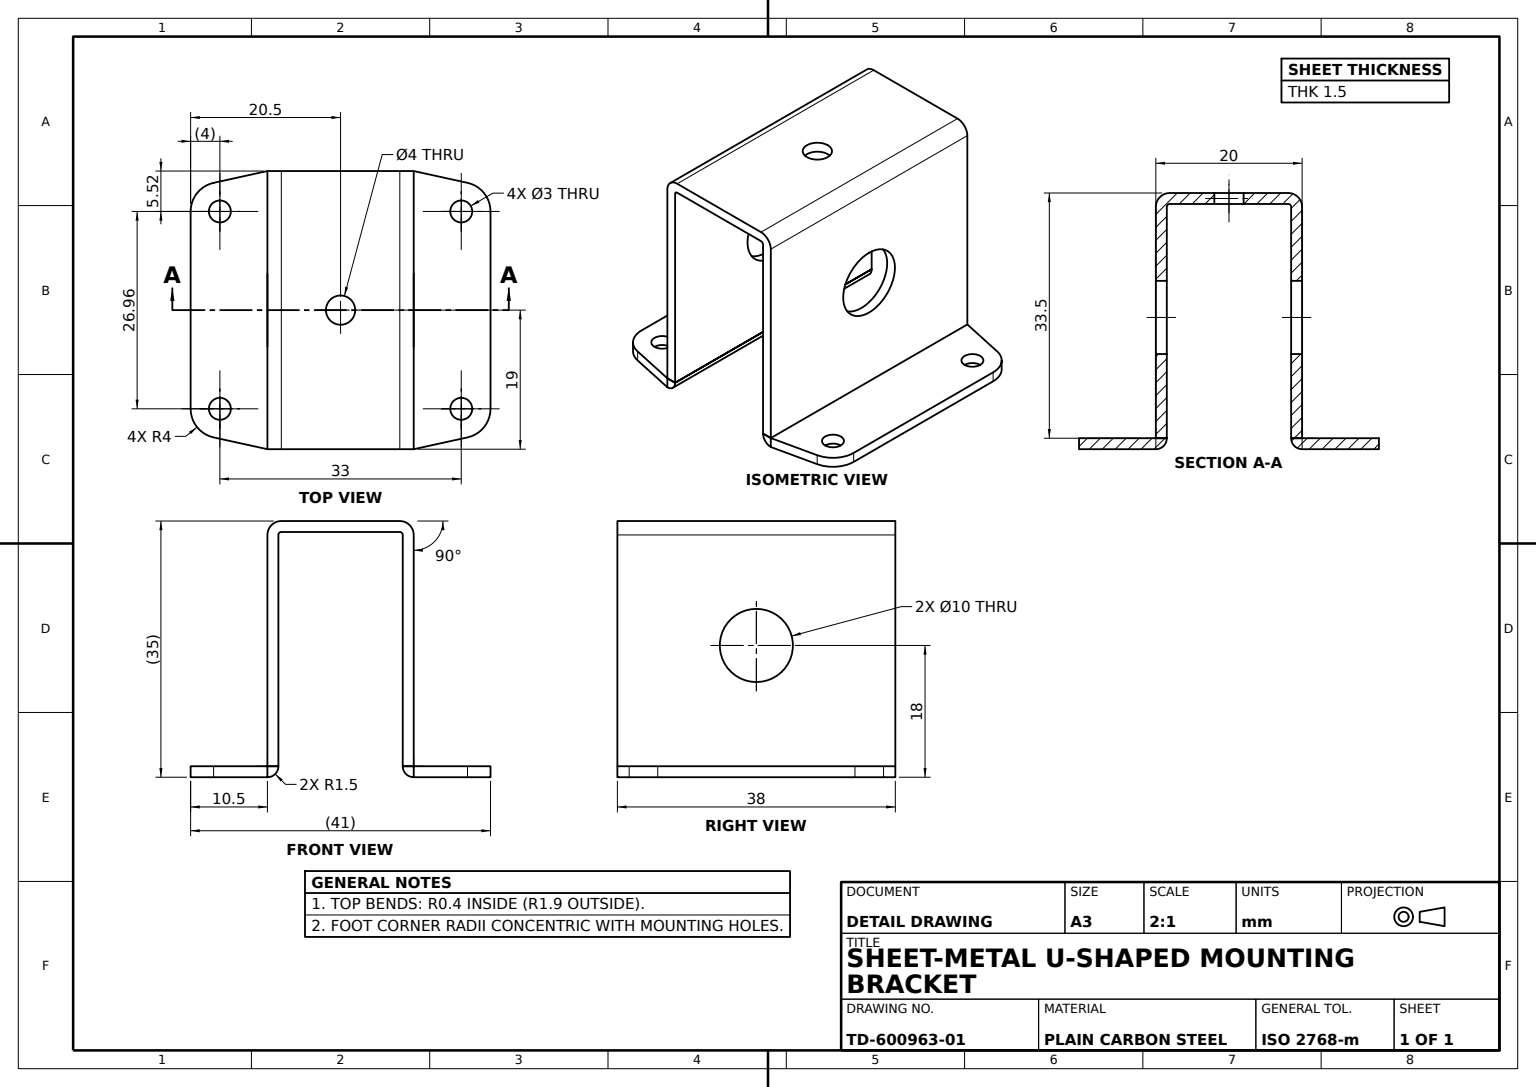
ISO-10303-21;
HEADER;
FILE_DESCRIPTION((''),'2;1');
FILE_NAME('','',(''),(''),'','','');
FILE_SCHEMA(('AUTOMOTIVE_DESIGN'));
ENDSEC;
DATA;
#1=APPLICATION_CONTEXT('');
#2=PRODUCT_CONTEXT('',#1,'mechanical');
#3=PRODUCT('','','',(#2));
#4=PRODUCT_DEFINITION_FORMATION('','',#3);
#5=PRODUCT_DEFINITION_CONTEXT('',#1,'design');
#6=PRODUCT_DEFINITION('','',#4,#5);
#7=PRODUCT_DEFINITION_SHAPE('','',#6);
#8=(LENGTH_UNIT()NAMED_UNIT(*)SI_UNIT(.MILLI.,.METRE.));
#9=(NAMED_UNIT(*)PLANE_ANGLE_UNIT()SI_UNIT($,.RADIAN.));
#10=(NAMED_UNIT(*)SI_UNIT($,.STERADIAN.)SOLID_ANGLE_UNIT());
#11=UNCERTAINTY_MEASURE_WITH_UNIT(LENGTH_MEASURE(1.E-05),#8,'distance_accuracy_value','');
#12=(GEOMETRIC_REPRESENTATION_CONTEXT(3)GLOBAL_UNCERTAINTY_ASSIGNED_CONTEXT((#11))GLOBAL_UNIT_ASSIGNED_CONTEXT((#8,#9,#10))REPRESENTATION_CONTEXT('',''));
#13=CARTESIAN_POINT('',(-15.,-33.5,13.481351));
#14=VERTEX_POINT('',#13);
#15=CARTESIAN_POINT('',(-18.,-33.5,13.481351));
#16=VERTEX_POINT('',#15);
#17=CARTESIAN_POINT('',(-16.5,-33.5,13.481351));
#18=DIRECTION('',(0.,-1.,0.));
#19=DIRECTION('',(1.,0.,0.));
#20=AXIS2_PLACEMENT_3D('',#17,#18,#19);
#21=CIRCLE('',#20,1.5);
#22=EDGE_CURVE('',#14,#16,#21,.T.);
#23=ORIENTED_EDGE('',*,*,#22,.F.);
#24=CARTESIAN_POINT('',(-15.,-35.,13.481351));
#25=VERTEX_POINT('',#24);
#26=DIRECTION('',(0.,1.,0.));
#27=VECTOR('',#26,1000.);
#28=LINE('',#24,#27);
#29=EDGE_CURVE('',#25,#14,#28,.T.);
#30=ORIENTED_EDGE('',*,*,#29,.F.);
#31=CARTESIAN_POINT('',(-18.,-35.,13.481351));
#32=VERTEX_POINT('',#31);
#33=CARTESIAN_POINT('',(-16.5,-35.,13.481351));
#34=AXIS2_PLACEMENT_3D('',#33,#18,#19);
#35=CIRCLE('',#34,1.5);
#36=EDGE_CURVE('',#25,#32,#35,.T.);
#37=ORIENTED_EDGE('',*,*,#36,.T.);
#38=LINE('',#31,#27);
#39=EDGE_CURVE('',#32,#16,#38,.T.);
#40=ORIENTED_EDGE('',*,*,#39,.T.);
#41=EDGE_LOOP('',(#23,#30,#37,#40));
#42=FACE_OUTER_BOUND('',#41,.T.);
#43=DIRECTION('',(-1.,0.,0.));
#44=AXIS2_PLACEMENT_3D('',#33,#26,#43);
#45=CYLINDRICAL_SURFACE('',#44,1.5);
#46=ADVANCED_FACE('',(#42),#45,.F.);
#47=CARTESIAN_POINT('',(-10.,-35.,19.));
#48=VERTEX_POINT('',#47);
#49=CARTESIAN_POINT('',(-10.,-33.5,19.));
#50=VERTEX_POINT('',#49);
#51=LINE('',#47,#27);
#52=EDGE_CURVE('',#48,#50,#51,.T.);
#53=ORIENTED_EDGE('',*,*,#52,.F.);
#54=CARTESIAN_POINT('',(-8.5,-33.5,19.));
#55=VERTEX_POINT('',#54);
#56=DIRECTION('',(0.,0.,1.));
#57=AXIS2_PLACEMENT_3D('',#49,#56,#26);
#58=CIRCLE('',#57,1.5);
#59=EDGE_CURVE('',#48,#55,#58,.T.);
#60=ORIENTED_EDGE('',*,*,#59,.T.);
#61=VECTOR('',#43,1000.);
#62=LINE('',#49,#61);
#63=EDGE_CURVE('',#55,#50,#62,.T.);
#64=ORIENTED_EDGE('',*,*,#63,.T.);
#65=EDGE_LOOP('',(#53,#60,#64));
#66=FACE_OUTER_BOUND('',#65,.T.);
#67=DIRECTION('',(0.,0.,-1.));
#68=AXIS2_PLACEMENT_3D('',#47,#67,#26);
#69=PLANE('',#68);
#70=ADVANCED_FACE('',(#66),#69,.F.);
#71=CARTESIAN_POINT('',(-17.355897,-35.,-17.388708));
#72=VERTEX_POINT('',#71);
#73=CARTESIAN_POINT('',(-17.355897,-33.5,-17.388708));
#74=VERTEX_POINT('',#73);
#75=LINE('',#71,#27);
#76=EDGE_CURVE('',#72,#74,#75,.T.);
#77=ORIENTED_EDGE('',*,*,#76,.F.);
#78=CARTESIAN_POINT('',(-20.5,-35.,-13.481351));
#79=VERTEX_POINT('',#78);
#80=CARTESIAN_POINT('',(-16.5,-35.,-13.481351));
#81=AXIS2_PLACEMENT_3D('',#80,#18,#19);
#82=CIRCLE('',#81,4.);
#83=EDGE_CURVE('',#79,#72,#82,.T.);
#84=ORIENTED_EDGE('',*,*,#83,.F.);
#85=CARTESIAN_POINT('',(-20.5,-33.5,-13.481351));
#86=VERTEX_POINT('',#85);
#87=LINE('',#78,#27);
#88=EDGE_CURVE('',#79,#86,#87,.T.);
#89=ORIENTED_EDGE('',*,*,#88,.T.);
#90=CARTESIAN_POINT('',(-16.5,-33.5,-13.481351));
#91=AXIS2_PLACEMENT_3D('',#90,#18,#19);
#92=CIRCLE('',#91,4.);
#93=EDGE_CURVE('',#86,#74,#92,.T.);
#94=ORIENTED_EDGE('',*,*,#93,.T.);
#95=EDGE_LOOP('',(#77,#84,#89,#94));
#96=FACE_OUTER_BOUND('',#95,.T.);
#97=AXIS2_PLACEMENT_3D('',#80,#26,#43);
#98=CYLINDRICAL_SURFACE('',#97,4.);
#99=ADVANCED_FACE('',(#96),#98,.T.);
#100=CARTESIAN_POINT('',(-18.,-33.5,-13.481351));
#101=VERTEX_POINT('',#100);
#102=CARTESIAN_POINT('',(-15.,-33.5,-13.481351));
#103=VERTEX_POINT('',#102);
#104=CIRCLE('',#91,1.5);
#105=EDGE_CURVE('',#101,#103,#104,.T.);
#106=ORIENTED_EDGE('',*,*,#105,.T.);
#107=EDGE_CURVE('',#103,#101,#104,.T.);
#108=ORIENTED_EDGE('',*,*,#107,.T.);
#109=EDGE_LOOP('',(#106,#108));
#110=FACE_BOUND('',#109,.T.);
#111=EDGE_CURVE('',#16,#14,#21,.T.);
#112=ORIENTED_EDGE('',*,*,#111,.T.);
#113=ORIENTED_EDGE('',*,*,#22,.T.);
#114=EDGE_LOOP('',(#112,#113));
#115=FACE_BOUND('',#114,.T.);
#116=CARTESIAN_POINT('',(-20.5,-33.5,13.481351));
#117=VERTEX_POINT('',#116);
#118=VECTOR('',#67,1000.);
#119=LINE('',#116,#118);
#120=EDGE_CURVE('',#117,#86,#119,.T.);
#121=ORIENTED_EDGE('',*,*,#120,.F.);
#122=CARTESIAN_POINT('',(-17.355897,-33.5,17.388708));
#123=VERTEX_POINT('',#122);
#124=AXIS2_PLACEMENT_3D('',#17,#18,#43);
#125=CIRCLE('',#124,4.);
#126=EDGE_CURVE('',#123,#117,#125,.T.);
#127=ORIENTED_EDGE('',*,*,#126,.F.);
#128=DIRECTION('',(-0.976839286,0.,-0.21397432));
#129=VECTOR('',#128,1000.);
#130=LINE('',#49,#129);
#131=EDGE_CURVE('',#50,#123,#130,.T.);
#132=ORIENTED_EDGE('',*,*,#131,.F.);
#133=ORIENTED_EDGE('',*,*,#63,.F.);
#134=CARTESIAN_POINT('',(-8.5,-33.5,-19.));
#135=VERTEX_POINT('',#134);
#136=VECTOR('',#56,1000.);
#137=LINE('',#54,#136);
#138=EDGE_CURVE('',#135,#55,#137,.T.);
#139=ORIENTED_EDGE('',*,*,#138,.F.);
#140=CARTESIAN_POINT('',(-10.,-33.5,-19.));
#141=VERTEX_POINT('',#140);
#142=VECTOR('',#19,1000.);
#143=LINE('',#140,#142);
#144=EDGE_CURVE('',#141,#135,#143,.T.);
#145=ORIENTED_EDGE('',*,*,#144,.F.);
#146=DIRECTION('',(0.976839286,0.,-0.21397432));
#147=VECTOR('',#146,1000.);
#148=LINE('',#73,#147);
#149=EDGE_CURVE('',#74,#141,#148,.T.);
#150=ORIENTED_EDGE('',*,*,#149,.F.);
#151=ORIENTED_EDGE('',*,*,#93,.F.);
#152=EDGE_LOOP('',(#121,#127,#132,#133,#139,#145,#150,#151));
#153=FACE_OUTER_BOUND('',#152,.T.);
#154=PLANE('',#91);
#155=ADVANCED_FACE('',(#110,#115,#153),#154,.F.);
#156=ORIENTED_EDGE('',*,*,#52,.T.);
#157=ORIENTED_EDGE('',*,*,#131,.T.);
#158=CARTESIAN_POINT('',(-17.355897,-35.,17.388708));
#159=VERTEX_POINT('',#158);
#160=LINE('',#158,#27);
#161=EDGE_CURVE('',#159,#123,#160,.T.);
#162=ORIENTED_EDGE('',*,*,#161,.F.);
#163=LINE('',#47,#129);
#164=EDGE_CURVE('',#48,#159,#163,.T.);
#165=ORIENTED_EDGE('',*,*,#164,.F.);
#166=EDGE_LOOP('',(#156,#157,#162,#165));
#167=FACE_OUTER_BOUND('',#166,.T.);
#168=DIRECTION('',(0.21397432,0.,-0.976839286));
#169=AXIS2_PLACEMENT_3D('',#47,#168,#128);
#170=PLANE('',#169);
#171=ADVANCED_FACE('',(#167),#170,.F.);
#172=ORIENTED_EDGE('',*,*,#138,.T.);
#173=ORIENTED_EDGE('',*,*,#59,.F.);
#174=CARTESIAN_POINT('',(-10.,-35.,-19.));
#175=VERTEX_POINT('',#174);
#176=LINE('',#47,#136);
#177=EDGE_CURVE('',#175,#48,#176,.T.);
#178=ORIENTED_EDGE('',*,*,#177,.F.);
#179=AXIS2_PLACEMENT_3D('',#140,#67,#18);
#180=CIRCLE('',#179,1.5);
#181=EDGE_CURVE('',#135,#175,#180,.T.);
#182=ORIENTED_EDGE('',*,*,#181,.F.);
#183=EDGE_LOOP('',(#172,#173,#178,#182));
#184=FACE_OUTER_BOUND('',#183,.T.);
#185=CARTESIAN_POINT('',(-10.,-33.5,-13.481351));
#186=AXIS2_PLACEMENT_3D('',#185,#67,#26);
#187=CYLINDRICAL_SURFACE('',#186,1.5);
#188=ADVANCED_FACE('',(#184),#187,.T.);
#189=ORIENTED_EDGE('',*,*,#161,.T.);
#190=ORIENTED_EDGE('',*,*,#126,.T.);
#191=CARTESIAN_POINT('',(-20.5,-35.,13.481351));
#192=VERTEX_POINT('',#191);
#193=LINE('',#191,#27);
#194=EDGE_CURVE('',#192,#117,#193,.T.);
#195=ORIENTED_EDGE('',*,*,#194,.F.);
#196=AXIS2_PLACEMENT_3D('',#33,#18,#43);
#197=CIRCLE('',#196,4.);
#198=EDGE_CURVE('',#159,#192,#197,.T.);
#199=ORIENTED_EDGE('',*,*,#198,.F.);
#200=EDGE_LOOP('',(#189,#190,#195,#199));
#201=FACE_OUTER_BOUND('',#200,.T.);
#202=CYLINDRICAL_SURFACE('',#44,4.);
#203=ADVANCED_FACE('',(#201),#202,.T.);
#204=ORIENTED_EDGE('',*,*,#144,.T.);
#205=ORIENTED_EDGE('',*,*,#181,.T.);
#206=LINE('',#174,#27);
#207=EDGE_CURVE('',#175,#141,#206,.T.);
#208=ORIENTED_EDGE('',*,*,#207,.T.);
#209=EDGE_LOOP('',(#204,#205,#208));
#210=FACE_OUTER_BOUND('',#209,.T.);
#211=AXIS2_PLACEMENT_3D('',#174,#56,#18);
#212=PLANE('',#211);
#213=ADVANCED_FACE('',(#210),#212,.F.);
#214=LINE('',#71,#147);
#215=EDGE_CURVE('',#72,#175,#214,.T.);
#216=ORIENTED_EDGE('',*,*,#215,.F.);
#217=ORIENTED_EDGE('',*,*,#76,.T.);
#218=ORIENTED_EDGE('',*,*,#149,.T.);
#219=ORIENTED_EDGE('',*,*,#207,.F.);
#220=EDGE_LOOP('',(#216,#217,#218,#219));
#221=FACE_OUTER_BOUND('',#220,.T.);
#222=DIRECTION('',(0.21397432,0.,0.976839286));
#223=AXIS2_PLACEMENT_3D('',#71,#222,#146);
#224=PLANE('',#223);
#225=ADVANCED_FACE('',(#221),#224,.F.);
#226=ORIENTED_EDGE('',*,*,#29,.T.);
#227=ORIENTED_EDGE('',*,*,#111,.F.);
#228=ORIENTED_EDGE('',*,*,#39,.F.);
#229=EDGE_CURVE('',#32,#25,#35,.T.);
#230=ORIENTED_EDGE('',*,*,#229,.T.);
#231=EDGE_LOOP('',(#226,#227,#228,#230));
#232=FACE_OUTER_BOUND('',#231,.T.);
#233=ADVANCED_FACE('',(#232),#45,.F.);
#234=ORIENTED_EDGE('',*,*,#120,.T.);
#235=ORIENTED_EDGE('',*,*,#88,.F.);
#236=LINE('',#191,#118);
#237=EDGE_CURVE('',#192,#79,#236,.T.);
#238=ORIENTED_EDGE('',*,*,#237,.F.);
#239=ORIENTED_EDGE('',*,*,#194,.T.);
#240=EDGE_LOOP('',(#234,#235,#238,#239));
#241=FACE_OUTER_BOUND('',#240,.T.);
#242=AXIS2_PLACEMENT_3D('',#191,#19,#26);
#243=PLANE('',#242);
#244=ADVANCED_FACE('',(#241),#243,.F.);
#245=ORIENTED_EDGE('',*,*,#105,.F.);
#246=CARTESIAN_POINT('',(-18.,-35.,-13.481351));
#247=VERTEX_POINT('',#246);
#248=LINE('',#246,#27);
#249=EDGE_CURVE('',#247,#101,#248,.T.);
#250=ORIENTED_EDGE('',*,*,#249,.F.);
#251=CARTESIAN_POINT('',(-15.,-35.,-13.481351));
#252=VERTEX_POINT('',#251);
#253=CIRCLE('',#81,1.5);
#254=EDGE_CURVE('',#247,#252,#253,.T.);
#255=ORIENTED_EDGE('',*,*,#254,.T.);
#256=LINE('',#251,#27);
#257=EDGE_CURVE('',#252,#103,#256,.T.);
#258=ORIENTED_EDGE('',*,*,#257,.T.);
#259=EDGE_LOOP('',(#245,#250,#255,#258));
#260=FACE_OUTER_BOUND('',#259,.T.);
#261=CYLINDRICAL_SURFACE('',#97,1.5);
#262=ADVANCED_FACE('',(#260),#261,.F.);
#263=ORIENTED_EDGE('',*,*,#257,.F.);
#264=EDGE_CURVE('',#252,#247,#253,.T.);
#265=ORIENTED_EDGE('',*,*,#264,.T.);
#266=ORIENTED_EDGE('',*,*,#249,.T.);
#267=ORIENTED_EDGE('',*,*,#107,.F.);
#268=EDGE_LOOP('',(#263,#265,#266,#267));
#269=FACE_OUTER_BOUND('',#268,.T.);
#270=ADVANCED_FACE('',(#269),#261,.F.);
#271=ORIENTED_EDGE('',*,*,#36,.F.);
#272=ORIENTED_EDGE('',*,*,#229,.F.);
#273=EDGE_LOOP('',(#271,#272));
#274=FACE_BOUND('',#273,.T.);
#275=ORIENTED_EDGE('',*,*,#198,.T.);
#276=ORIENTED_EDGE('',*,*,#237,.T.);
#277=ORIENTED_EDGE('',*,*,#83,.T.);
#278=ORIENTED_EDGE('',*,*,#215,.T.);
#279=ORIENTED_EDGE('',*,*,#177,.T.);
#280=ORIENTED_EDGE('',*,*,#164,.T.);
#281=EDGE_LOOP('',(#275,#276,#277,#278,#279,#280));
#282=FACE_OUTER_BOUND('',#281,.T.);
#283=ORIENTED_EDGE('',*,*,#254,.F.);
#284=ORIENTED_EDGE('',*,*,#264,.F.);
#285=EDGE_LOOP('',(#283,#284));
#286=FACE_BOUND('',#285,.T.);
#287=PLANE('',#81);
#288=ADVANCED_FACE('',(#274,#282,#286),#287,.T.);
#289=CLOSED_SHELL('',(#46,#70,#99,#155,#171,#188,#203,#213,#225,#233,#244,#262,#270,#288));
#290=MANIFOLD_SOLID_BREP('',#289);
#291=CARTESIAN_POINT('',(10.,-35.,-19.));
#292=VERTEX_POINT('',#291);
#293=CARTESIAN_POINT('',(10.,-33.5,-19.));
#294=VERTEX_POINT('',#293);
#295=LINE('',#291,#27);
#296=EDGE_CURVE('',#292,#294,#295,.T.);
#297=ORIENTED_EDGE('',*,*,#296,.F.);
#298=CARTESIAN_POINT('',(8.5,-33.5,-19.));
#299=VERTEX_POINT('',#298);
#300=AXIS2_PLACEMENT_3D('',#293,#56,#18);
#301=CIRCLE('',#300,1.5);
#302=EDGE_CURVE('',#299,#292,#301,.T.);
#303=ORIENTED_EDGE('',*,*,#302,.F.);
#304=LINE('',#293,#61);
#305=EDGE_CURVE('',#294,#299,#304,.T.);
#306=ORIENTED_EDGE('',*,*,#305,.F.);
#307=EDGE_LOOP('',(#297,#303,#306));
#308=FACE_OUTER_BOUND('',#307,.T.);
#309=AXIS2_PLACEMENT_3D('',#291,#56,#18);
#310=PLANE('',#309);
#311=ADVANCED_FACE('',(#308),#310,.F.);
#312=CARTESIAN_POINT('',(18.,-33.5,-13.481351));
#313=VERTEX_POINT('',#312);
#314=CARTESIAN_POINT('',(15.,-33.5,-13.481351));
#315=VERTEX_POINT('',#314);
#316=CARTESIAN_POINT('',(16.5,-33.5,-13.481351));
#317=AXIS2_PLACEMENT_3D('',#316,#26,#43);
#318=CIRCLE('',#317,1.5);
#319=EDGE_CURVE('',#313,#315,#318,.T.);
#320=ORIENTED_EDGE('',*,*,#319,.F.);
#321=EDGE_CURVE('',#315,#313,#318,.T.);
#322=ORIENTED_EDGE('',*,*,#321,.F.);
#323=EDGE_LOOP('',(#320,#322));
#324=FACE_BOUND('',#323,.T.);
#325=CARTESIAN_POINT('',(15.,-33.5,13.481351));
#326=VERTEX_POINT('',#325);
#327=CARTESIAN_POINT('',(18.,-33.5,13.481351));
#328=VERTEX_POINT('',#327);
#329=CARTESIAN_POINT('',(16.5,-33.5,13.481351));
#330=AXIS2_PLACEMENT_3D('',#329,#26,#43);
#331=CIRCLE('',#330,1.5);
#332=EDGE_CURVE('',#326,#328,#331,.T.);
#333=ORIENTED_EDGE('',*,*,#332,.F.);
#334=EDGE_CURVE('',#328,#326,#331,.T.);
#335=ORIENTED_EDGE('',*,*,#334,.F.);
#336=EDGE_LOOP('',(#333,#335));
#337=FACE_BOUND('',#336,.T.);
#338=CARTESIAN_POINT('',(20.5,-33.5,-13.481351));
#339=VERTEX_POINT('',#338);
#340=CARTESIAN_POINT('',(17.355897,-33.5,-17.388708));
#341=VERTEX_POINT('',#340);
#342=CIRCLE('',#317,4.);
#343=EDGE_CURVE('',#339,#341,#342,.T.);
#344=ORIENTED_EDGE('',*,*,#343,.T.);
#345=LINE('',#340,#129);
#346=EDGE_CURVE('',#341,#294,#345,.T.);
#347=ORIENTED_EDGE('',*,*,#346,.T.);
#348=ORIENTED_EDGE('',*,*,#305,.T.);
#349=CARTESIAN_POINT('',(8.5,-33.5,19.));
#350=VERTEX_POINT('',#349);
#351=LINE('',#349,#136);
#352=EDGE_CURVE('',#299,#350,#351,.T.);
#353=ORIENTED_EDGE('',*,*,#352,.T.);
#354=CARTESIAN_POINT('',(10.,-33.5,19.));
#355=VERTEX_POINT('',#354);
#356=LINE('',#354,#142);
#357=EDGE_CURVE('',#350,#355,#356,.T.);
#358=ORIENTED_EDGE('',*,*,#357,.T.);
#359=CARTESIAN_POINT('',(17.355897,-33.5,17.388708));
#360=VERTEX_POINT('',#359);
#361=LINE('',#354,#147);
#362=EDGE_CURVE('',#355,#360,#361,.T.);
#363=ORIENTED_EDGE('',*,*,#362,.T.);
#364=CARTESIAN_POINT('',(20.5,-33.5,13.481351));
#365=VERTEX_POINT('',#364);
#366=AXIS2_PLACEMENT_3D('',#329,#26,#19);
#367=CIRCLE('',#366,4.);
#368=EDGE_CURVE('',#360,#365,#367,.T.);
#369=ORIENTED_EDGE('',*,*,#368,.T.);
#370=LINE('',#364,#118);
#371=EDGE_CURVE('',#365,#339,#370,.T.);
#372=ORIENTED_EDGE('',*,*,#371,.T.);
#373=EDGE_LOOP('',(#344,#347,#348,#353,#358,#363,#369,#372));
#374=FACE_OUTER_BOUND('',#373,.T.);
#375=AXIS2_PLACEMENT_3D('',#316,#18,#43);
#376=PLANE('',#375);
#377=ADVANCED_FACE('',(#324,#337,#374),#376,.F.);
#378=CARTESIAN_POINT('',(17.355897,-35.,17.388708));
#379=VERTEX_POINT('',#378);
#380=LINE('',#378,#27);
#381=EDGE_CURVE('',#379,#360,#380,.T.);
#382=ORIENTED_EDGE('',*,*,#381,.F.);
#383=CARTESIAN_POINT('',(20.5,-35.,13.481351));
#384=VERTEX_POINT('',#383);
#385=CARTESIAN_POINT('',(16.5,-35.,13.481351));
#386=AXIS2_PLACEMENT_3D('',#385,#26,#19);
#387=CIRCLE('',#386,4.);
#388=EDGE_CURVE('',#379,#384,#387,.T.);
#389=ORIENTED_EDGE('',*,*,#388,.T.);
#390=LINE('',#383,#27);
#391=EDGE_CURVE('',#384,#365,#390,.T.);
#392=ORIENTED_EDGE('',*,*,#391,.T.);
#393=ORIENTED_EDGE('',*,*,#368,.F.);
#394=EDGE_LOOP('',(#382,#389,#392,#393));
#395=FACE_OUTER_BOUND('',#394,.T.);
#396=CYLINDRICAL_SURFACE('',#386,4.);
#397=ADVANCED_FACE('',(#395),#396,.T.);
#398=CARTESIAN_POINT('',(17.355897,-35.,-17.388708));
#399=VERTEX_POINT('',#398);
#400=LINE('',#398,#129);
#401=EDGE_CURVE('',#399,#292,#400,.T.);
#402=ORIENTED_EDGE('',*,*,#401,.T.);
#403=ORIENTED_EDGE('',*,*,#296,.T.);
#404=ORIENTED_EDGE('',*,*,#346,.F.);
#405=LINE('',#398,#27);
#406=EDGE_CURVE('',#399,#341,#405,.T.);
#407=ORIENTED_EDGE('',*,*,#406,.F.);
#408=EDGE_LOOP('',(#402,#403,#404,#407));
#409=FACE_OUTER_BOUND('',#408,.T.);
#410=DIRECTION('',(-0.21397432,0.,0.976839286));
#411=AXIS2_PLACEMENT_3D('',#398,#410,#128);
#412=PLANE('',#411);
#413=ADVANCED_FACE('',(#409),#412,.F.);
#414=CARTESIAN_POINT('',(20.5,-35.,-13.481351));
#415=VERTEX_POINT('',#414);
#416=LINE('',#414,#27);
#417=EDGE_CURVE('',#415,#339,#416,.T.);
#418=ORIENTED_EDGE('',*,*,#417,.T.);
#419=ORIENTED_EDGE('',*,*,#371,.F.);
#420=ORIENTED_EDGE('',*,*,#391,.F.);
#421=LINE('',#383,#118);
#422=EDGE_CURVE('',#384,#415,#421,.T.);
#423=ORIENTED_EDGE('',*,*,#422,.T.);
#424=EDGE_LOOP('',(#418,#419,#420,#423));
#425=FACE_OUTER_BOUND('',#424,.T.);
#426=AXIS2_PLACEMENT_3D('',#383,#43,#26);
#427=PLANE('',#426);
#428=ADVANCED_FACE('',(#425),#427,.F.);
#429=CARTESIAN_POINT('',(15.,-35.,-13.481351));
#430=VERTEX_POINT('',#429);
#431=CARTESIAN_POINT('',(18.,-35.,-13.481351));
#432=VERTEX_POINT('',#431);
#433=CARTESIAN_POINT('',(16.5,-35.,-13.481351));
#434=AXIS2_PLACEMENT_3D('',#433,#26,#43);
#435=CIRCLE('',#434,1.5);
#436=EDGE_CURVE('',#430,#432,#435,.T.);
#437=ORIENTED_EDGE('',*,*,#436,.F.);
#438=LINE('',#429,#27);
#439=EDGE_CURVE('',#430,#315,#438,.T.);
#440=ORIENTED_EDGE('',*,*,#439,.T.);
#441=ORIENTED_EDGE('',*,*,#321,.T.);
#442=LINE('',#431,#27);
#443=EDGE_CURVE('',#432,#313,#442,.T.);
#444=ORIENTED_EDGE('',*,*,#443,.F.);
#445=EDGE_LOOP('',(#437,#440,#441,#444));
#446=FACE_OUTER_BOUND('',#445,.T.);
#447=AXIS2_PLACEMENT_3D('',#433,#26,#19);
#448=CYLINDRICAL_SURFACE('',#447,1.5);
#449=ADVANCED_FACE('',(#446),#448,.F.);
#450=CARTESIAN_POINT('',(18.,-35.,13.481351));
#451=VERTEX_POINT('',#450);
#452=CARTESIAN_POINT('',(15.,-35.,13.481351));
#453=VERTEX_POINT('',#452);
#454=AXIS2_PLACEMENT_3D('',#385,#26,#43);
#455=CIRCLE('',#454,1.5);
#456=EDGE_CURVE('',#451,#453,#455,.T.);
#457=ORIENTED_EDGE('',*,*,#456,.F.);
#458=LINE('',#450,#27);
#459=EDGE_CURVE('',#451,#328,#458,.T.);
#460=ORIENTED_EDGE('',*,*,#459,.T.);
#461=ORIENTED_EDGE('',*,*,#334,.T.);
#462=LINE('',#452,#27);
#463=EDGE_CURVE('',#453,#326,#462,.T.);
#464=ORIENTED_EDGE('',*,*,#463,.F.);
#465=EDGE_LOOP('',(#457,#460,#461,#464));
#466=FACE_OUTER_BOUND('',#465,.T.);
#467=CYLINDRICAL_SURFACE('',#386,1.5);
#468=ADVANCED_FACE('',(#466),#467,.F.);
#469=ORIENTED_EDGE('',*,*,#343,.F.);
#470=ORIENTED_EDGE('',*,*,#417,.F.);
#471=CIRCLE('',#434,4.);
#472=EDGE_CURVE('',#415,#399,#471,.T.);
#473=ORIENTED_EDGE('',*,*,#472,.T.);
#474=ORIENTED_EDGE('',*,*,#406,.T.);
#475=EDGE_LOOP('',(#469,#470,#473,#474));
#476=FACE_OUTER_BOUND('',#475,.T.);
#477=CYLINDRICAL_SURFACE('',#447,4.);
#478=ADVANCED_FACE('',(#476),#477,.T.);
#479=ORIENTED_EDGE('',*,*,#456,.T.);
#480=EDGE_CURVE('',#453,#451,#455,.T.);
#481=ORIENTED_EDGE('',*,*,#480,.T.);
#482=EDGE_LOOP('',(#479,#481));
#483=FACE_BOUND('',#482,.T.);
#484=ORIENTED_EDGE('',*,*,#388,.F.);
#485=CARTESIAN_POINT('',(10.,-35.,19.));
#486=VERTEX_POINT('',#485);
#487=LINE('',#485,#147);
#488=EDGE_CURVE('',#486,#379,#487,.T.);
#489=ORIENTED_EDGE('',*,*,#488,.F.);
#490=LINE('',#485,#136);
#491=EDGE_CURVE('',#292,#486,#490,.T.);
#492=ORIENTED_EDGE('',*,*,#491,.F.);
#493=ORIENTED_EDGE('',*,*,#401,.F.);
#494=ORIENTED_EDGE('',*,*,#472,.F.);
#495=ORIENTED_EDGE('',*,*,#422,.F.);
#496=EDGE_LOOP('',(#484,#489,#492,#493,#494,#495));
#497=FACE_OUTER_BOUND('',#496,.T.);
#498=ORIENTED_EDGE('',*,*,#436,.T.);
#499=EDGE_CURVE('',#432,#430,#435,.T.);
#500=ORIENTED_EDGE('',*,*,#499,.T.);
#501=EDGE_LOOP('',(#498,#500));
#502=FACE_BOUND('',#501,.T.);
#503=AXIS2_PLACEMENT_3D('',#433,#18,#43);
#504=PLANE('',#503);
#505=ADVANCED_FACE('',(#483,#497,#502),#504,.T.);
#506=ORIENTED_EDGE('',*,*,#319,.T.);
#507=ORIENTED_EDGE('',*,*,#439,.F.);
#508=ORIENTED_EDGE('',*,*,#499,.F.);
#509=ORIENTED_EDGE('',*,*,#443,.T.);
#510=EDGE_LOOP('',(#506,#507,#508,#509));
#511=FACE_OUTER_BOUND('',#510,.T.);
#512=ADVANCED_FACE('',(#511),#448,.F.);
#513=ORIENTED_EDGE('',*,*,#463,.T.);
#514=ORIENTED_EDGE('',*,*,#332,.T.);
#515=ORIENTED_EDGE('',*,*,#459,.F.);
#516=ORIENTED_EDGE('',*,*,#480,.F.);
#517=EDGE_LOOP('',(#513,#514,#515,#516));
#518=FACE_OUTER_BOUND('',#517,.T.);
#519=ADVANCED_FACE('',(#518),#467,.F.);
#520=AXIS2_PLACEMENT_3D('',#354,#67,#26);
#521=CIRCLE('',#520,1.5);
#522=EDGE_CURVE('',#486,#350,#521,.T.);
#523=ORIENTED_EDGE('',*,*,#522,.T.);
#524=ORIENTED_EDGE('',*,*,#352,.F.);
#525=ORIENTED_EDGE('',*,*,#302,.T.);
#526=ORIENTED_EDGE('',*,*,#491,.T.);
#527=EDGE_LOOP('',(#523,#524,#525,#526));
#528=FACE_OUTER_BOUND('',#527,.T.);
#529=CARTESIAN_POINT('',(10.,-33.5,-13.481351));
#530=AXIS2_PLACEMENT_3D('',#529,#67,#26);
#531=CYLINDRICAL_SURFACE('',#530,1.5);
#532=ADVANCED_FACE('',(#528),#531,.T.);
#533=ORIENTED_EDGE('',*,*,#381,.T.);
#534=ORIENTED_EDGE('',*,*,#362,.F.);
#535=LINE('',#485,#27);
#536=EDGE_CURVE('',#486,#355,#535,.T.);
#537=ORIENTED_EDGE('',*,*,#536,.F.);
#538=ORIENTED_EDGE('',*,*,#488,.T.);
#539=EDGE_LOOP('',(#533,#534,#537,#538));
#540=FACE_OUTER_BOUND('',#539,.T.);
#541=DIRECTION('',(-0.21397432,0.,-0.976839286));
#542=AXIS2_PLACEMENT_3D('',#485,#541,#146);
#543=PLANE('',#542);
#544=ADVANCED_FACE('',(#540),#543,.F.);
#545=ORIENTED_EDGE('',*,*,#357,.F.);
#546=ORIENTED_EDGE('',*,*,#522,.F.);
#547=ORIENTED_EDGE('',*,*,#536,.T.);
#548=EDGE_LOOP('',(#545,#546,#547));
#549=FACE_OUTER_BOUND('',#548,.T.);
#550=AXIS2_PLACEMENT_3D('',#485,#67,#26);
#551=PLANE('',#550);
#552=ADVANCED_FACE('',(#549),#551,.F.);
#553=CLOSED_SHELL('',(#311,#377,#397,#413,#428,#449,#468,#478,#505,#512,#519,#532,#544,#552));
#554=MANIFOLD_SOLID_BREP('',#553);
#555=VERTEX_POINT('',#349);
#556=CARTESIAN_POINT('',(8.5,-1.9,19.));
#557=VERTEX_POINT('',#556);
#558=CARTESIAN_POINT('',(8.5,0.,19.));
#559=LINE('',#558,#27);
#560=EDGE_CURVE('',#555,#557,#559,.T.);
#561=ORIENTED_EDGE('',*,*,#560,.F.);
#562=VERTEX_POINT('',#354);
#563=LINE('',#354,#61);
#564=EDGE_CURVE('',#562,#555,#563,.T.);
#565=ORIENTED_EDGE('',*,*,#564,.F.);
#566=CARTESIAN_POINT('',(10.,-1.9,19.));
#567=VERTEX_POINT('',#566);
#568=LINE('',#354,#27);
#569=EDGE_CURVE('',#562,#567,#568,.T.);
#570=ORIENTED_EDGE('',*,*,#569,.T.);
#571=LINE('',#556,#142);
#572=EDGE_CURVE('',#557,#567,#571,.T.);
#573=ORIENTED_EDGE('',*,*,#572,.F.);
#574=EDGE_LOOP('',(#561,#565,#570,#573));
#575=FACE_OUTER_BOUND('',#574,.T.);
#576=AXIS2_PLACEMENT_3D('',#354,#56,#19);
#577=PLANE('',#576);
#578=ADVANCED_FACE('',(#575),#577,.T.);
#579=CARTESIAN_POINT('',(8.1,-1.5,-19.));
#580=VERTEX_POINT('',#579);
#581=CARTESIAN_POINT('',(8.5,-1.9,-19.));
#582=VERTEX_POINT('',#581);
#583=CARTESIAN_POINT('',(8.1,-1.9,-19.));
#584=AXIS2_PLACEMENT_3D('',#583,#67,#19);
#585=CIRCLE('',#584,0.4);
#586=EDGE_CURVE('',#580,#582,#585,.T.);
#587=ORIENTED_EDGE('',*,*,#586,.T.);
#588=LINE('',#581,#136);
#589=EDGE_CURVE('',#582,#557,#588,.T.);
#590=ORIENTED_EDGE('',*,*,#589,.T.);
#591=CARTESIAN_POINT('',(8.1,-1.5,19.));
#592=VERTEX_POINT('',#591);
#593=CARTESIAN_POINT('',(8.1,-1.9,19.));
#594=AXIS2_PLACEMENT_3D('',#593,#56,#19);
#595=CIRCLE('',#594,0.4);
#596=EDGE_CURVE('',#557,#592,#595,.T.);
#597=ORIENTED_EDGE('',*,*,#596,.T.);
#598=LINE('',#591,#118);
#599=EDGE_CURVE('',#592,#580,#598,.T.);
#600=ORIENTED_EDGE('',*,*,#599,.T.);
#601=EDGE_LOOP('',(#587,#590,#597,#600));
#602=FACE_OUTER_BOUND('',#601,.T.);
#603=CYLINDRICAL_SURFACE('',#594,0.4);
#604=ADVANCED_FACE('',(#602),#603,.F.);
#605=ORIENTED_EDGE('',*,*,#586,.F.);
#606=CARTESIAN_POINT('',(8.1,0.,-19.));
#607=VERTEX_POINT('',#606);
#608=LINE('',#579,#27);
#609=EDGE_CURVE('',#580,#607,#608,.T.);
#610=ORIENTED_EDGE('',*,*,#609,.T.);
#611=CARTESIAN_POINT('',(10.,-1.9,-19.));
#612=VERTEX_POINT('',#611);
#613=CIRCLE('',#584,1.9);
#614=EDGE_CURVE('',#607,#612,#613,.T.);
#615=ORIENTED_EDGE('',*,*,#614,.T.);
#616=LINE('',#611,#142);
#617=EDGE_CURVE('',#582,#612,#616,.T.);
#618=ORIENTED_EDGE('',*,*,#617,.F.);
#619=EDGE_LOOP('',(#605,#610,#615,#618));
#620=FACE_OUTER_BOUND('',#619,.T.);
#621=AXIS2_PLACEMENT_3D('',#583,#67,#43);
#622=PLANE('',#621);
#623=ADVANCED_FACE('',(#620),#622,.T.);
#624=LINE('',#611,#118);
#625=EDGE_CURVE('',#567,#612,#624,.T.);
#626=ORIENTED_EDGE('',*,*,#625,.T.);
#627=ORIENTED_EDGE('',*,*,#614,.F.);
#628=CARTESIAN_POINT('',(8.1,0.,19.));
#629=VERTEX_POINT('',#628);
#630=LINE('',#628,#118);
#631=EDGE_CURVE('',#629,#607,#630,.T.);
#632=ORIENTED_EDGE('',*,*,#631,.F.);
#633=CIRCLE('',#594,1.9);
#634=EDGE_CURVE('',#567,#629,#633,.T.);
#635=ORIENTED_EDGE('',*,*,#634,.F.);
#636=EDGE_LOOP('',(#626,#627,#632,#635));
#637=FACE_OUTER_BOUND('',#636,.T.);
#638=CYLINDRICAL_SURFACE('',#594,1.9);
#639=ADVANCED_FACE('',(#637),#638,.T.);
#640=CARTESIAN_POINT('',(0.,-1.5,2.));
#641=VERTEX_POINT('',#640);
#642=CARTESIAN_POINT('',(0.,0.,2.));
#643=VERTEX_POINT('',#642);
#644=CARTESIAN_POINT('',(0.,-10.,2.));
#645=LINE('',#644,#27);
#646=EDGE_CURVE('',#641,#643,#645,.T.);
#647=ORIENTED_EDGE('',*,*,#646,.F.);
#648=CARTESIAN_POINT('',(0.,-1.5,-2.));
#649=VERTEX_POINT('',#648);
#650=CARTESIAN_POINT('',(0.,-1.5,0.));
#651=AXIS2_PLACEMENT_3D('',#650,#26,#56);
#652=CIRCLE('',#651,2.);
#653=EDGE_CURVE('',#649,#641,#652,.T.);
#654=ORIENTED_EDGE('',*,*,#653,.F.);
#655=CARTESIAN_POINT('',(0.,0.,-2.));
#656=VERTEX_POINT('',#655);
#657=CARTESIAN_POINT('',(0.,-10.,-2.));
#658=LINE('',#657,#27);
#659=EDGE_CURVE('',#649,#656,#658,.T.);
#660=ORIENTED_EDGE('',*,*,#659,.T.);
#661=CARTESIAN_POINT('',(0.,0.,0.));
#662=AXIS2_PLACEMENT_3D('',#661,#26,#56);
#663=CIRCLE('',#662,2.);
#664=EDGE_CURVE('',#656,#643,#663,.T.);
#665=ORIENTED_EDGE('',*,*,#664,.T.);
#666=EDGE_LOOP('',(#647,#654,#660,#665));
#667=FACE_OUTER_BOUND('',#666,.T.);
#668=CARTESIAN_POINT('',(0.,-10.,0.));
#669=AXIS2_PLACEMENT_3D('',#668,#26,#56);
#670=CYLINDRICAL_SURFACE('',#669,2.);
#671=ADVANCED_FACE('',(#667),#670,.F.);
#672=ORIENTED_EDGE('',*,*,#599,.F.);
#673=CARTESIAN_POINT('',(-8.1,-1.5,19.));
#674=VERTEX_POINT('',#673);
#675=CARTESIAN_POINT('',(-10.,-1.5,19.));
#676=LINE('',#675,#142);
#677=EDGE_CURVE('',#674,#592,#676,.T.);
#678=ORIENTED_EDGE('',*,*,#677,.F.);
#679=CARTESIAN_POINT('',(-8.1,-1.5,-19.));
#680=VERTEX_POINT('',#679);
#681=LINE('',#679,#136);
#682=EDGE_CURVE('',#680,#674,#681,.T.);
#683=ORIENTED_EDGE('',*,*,#682,.F.);
#684=CARTESIAN_POINT('',(-10.,-1.5,-19.));
#685=LINE('',#684,#61);
#686=EDGE_CURVE('',#580,#680,#685,.T.);
#687=ORIENTED_EDGE('',*,*,#686,.F.);
#688=EDGE_LOOP('',(#672,#678,#683,#687));
#689=FACE_OUTER_BOUND('',#688,.T.);
#690=ORIENTED_EDGE('',*,*,#653,.T.);
#691=EDGE_CURVE('',#641,#649,#652,.T.);
#692=ORIENTED_EDGE('',*,*,#691,.T.);
#693=EDGE_LOOP('',(#690,#692));
#694=FACE_BOUND('',#693,.T.);
#695=PLANE('',#651);
#696=ADVANCED_FACE('',(#689,#694),#695,.F.);
#697=VERTEX_POINT('',#293);
#698=VERTEX_POINT('',#298);
#699=EDGE_CURVE('',#697,#698,#304,.T.);
#700=ORIENTED_EDGE('',*,*,#699,.T.);
#701=CARTESIAN_POINT('',(8.5,0.,-19.));
#702=VECTOR('',#18,1000.);
#703=LINE('',#701,#702);
#704=EDGE_CURVE('',#582,#698,#703,.T.);
#705=ORIENTED_EDGE('',*,*,#704,.F.);
#706=ORIENTED_EDGE('',*,*,#617,.T.);
#707=CARTESIAN_POINT('',(10.,-1.5,-19.));
#708=LINE('',#707,#702);
#709=EDGE_CURVE('',#612,#697,#708,.T.);
#710=ORIENTED_EDGE('',*,*,#709,.T.);
#711=EDGE_LOOP('',(#700,#705,#706,#710));
#712=FACE_OUTER_BOUND('',#711,.T.);
#713=AXIS2_PLACEMENT_3D('',#707,#67,#43);
#714=PLANE('',#713);
#715=ADVANCED_FACE('',(#712),#714,.T.);
#716=ORIENTED_EDGE('',*,*,#560,.T.);
#717=ORIENTED_EDGE('',*,*,#589,.F.);
#718=ORIENTED_EDGE('',*,*,#704,.T.);
#719=CARTESIAN_POINT('',(8.5,-33.5,0.));
#720=LINE('',#719,#136);
#721=EDGE_CURVE('',#698,#555,#720,.T.);
#722=ORIENTED_EDGE('',*,*,#721,.T.);
#723=EDGE_LOOP('',(#716,#717,#718,#722));
#724=FACE_OUTER_BOUND('',#723,.T.);
#725=CARTESIAN_POINT('',(8.5,-12.,0.));
#726=VERTEX_POINT('',#725);
#727=CARTESIAN_POINT('',(8.5,-22.,0.));
#728=VERTEX_POINT('',#727);
#729=CARTESIAN_POINT('',(8.5,-17.,0.));
#730=AXIS2_PLACEMENT_3D('',#729,#43,#18);
#731=CIRCLE('',#730,5.);
#732=EDGE_CURVE('',#726,#728,#731,.T.);
#733=ORIENTED_EDGE('',*,*,#732,.F.);
#734=EDGE_CURVE('',#728,#726,#731,.T.);
#735=ORIENTED_EDGE('',*,*,#734,.F.);
#736=EDGE_LOOP('',(#733,#735));
#737=FACE_BOUND('',#736,.T.);
#738=CARTESIAN_POINT('',(8.5,0.,0.));
#739=AXIS2_PLACEMENT_3D('',#738,#43,#18);
#740=PLANE('',#739);
#741=ADVANCED_FACE('',(#724,#737),#740,.T.);
#742=ORIENTED_EDGE('',*,*,#732,.T.);
#743=CARTESIAN_POINT('',(10.,-22.,0.));
#744=VERTEX_POINT('',#743);
#745=CARTESIAN_POINT('',(30.,-22.,0.));
#746=LINE('',#745,#61);
#747=EDGE_CURVE('',#744,#728,#746,.T.);
#748=ORIENTED_EDGE('',*,*,#747,.F.);
#749=CARTESIAN_POINT('',(10.,-12.,0.));
#750=VERTEX_POINT('',#749);
#751=CARTESIAN_POINT('',(10.,-17.,0.));
#752=AXIS2_PLACEMENT_3D('',#751,#43,#18);
#753=CIRCLE('',#752,5.);
#754=EDGE_CURVE('',#750,#744,#753,.T.);
#755=ORIENTED_EDGE('',*,*,#754,.F.);
#756=CARTESIAN_POINT('',(30.,-12.,0.));
#757=LINE('',#756,#61);
#758=EDGE_CURVE('',#750,#726,#757,.T.);
#759=ORIENTED_EDGE('',*,*,#758,.T.);
#760=EDGE_LOOP('',(#742,#748,#755,#759));
#761=FACE_OUTER_BOUND('',#760,.T.);
#762=CARTESIAN_POINT('',(30.,-17.,0.));
#763=AXIS2_PLACEMENT_3D('',#762,#43,#18);
#764=CYLINDRICAL_SURFACE('',#763,5.);
#765=ADVANCED_FACE('',(#761),#764,.F.);
#766=CARTESIAN_POINT('',(-8.5,-1.9,19.));
#767=VERTEX_POINT('',#766);
#768=CARTESIAN_POINT('',(-10.,-1.9,19.));
#769=VERTEX_POINT('',#768);
#770=LINE('',#768,#61);
#771=EDGE_CURVE('',#767,#769,#770,.T.);
#772=ORIENTED_EDGE('',*,*,#771,.F.);
#773=CARTESIAN_POINT('',(-8.1,-1.9,19.));
#774=AXIS2_PLACEMENT_3D('',#773,#56,#43);
#775=CIRCLE('',#774,0.4);
#776=EDGE_CURVE('',#674,#767,#775,.T.);
#777=ORIENTED_EDGE('',*,*,#776,.F.);
#778=CARTESIAN_POINT('',(-8.1,0.,19.));
#779=VERTEX_POINT('',#778);
#780=LINE('',#673,#27);
#781=EDGE_CURVE('',#674,#779,#780,.T.);
#782=ORIENTED_EDGE('',*,*,#781,.T.);
#783=CIRCLE('',#774,1.9);
#784=EDGE_CURVE('',#779,#769,#783,.T.);
#785=ORIENTED_EDGE('',*,*,#784,.T.);
#786=EDGE_LOOP('',(#772,#777,#782,#785));
#787=FACE_OUTER_BOUND('',#786,.T.);
#788=AXIS2_PLACEMENT_3D('',#773,#56,#19);
#789=PLANE('',#788);
#790=ADVANCED_FACE('',(#787),#789,.T.);
#791=ORIENTED_EDGE('',*,*,#609,.F.);
#792=ORIENTED_EDGE('',*,*,#686,.T.);
#793=CARTESIAN_POINT('',(-8.1,0.,-19.));
#794=VERTEX_POINT('',#793);
#795=LINE('',#679,#27);
#796=EDGE_CURVE('',#680,#794,#795,.T.);
#797=ORIENTED_EDGE('',*,*,#796,.T.);
#798=CARTESIAN_POINT('',(-10.,0.,-19.));
#799=LINE('',#798,#61);
#800=EDGE_CURVE('',#607,#794,#799,.T.);
#801=ORIENTED_EDGE('',*,*,#800,.F.);
#802=EDGE_LOOP('',(#791,#792,#797,#801));
#803=FACE_OUTER_BOUND('',#802,.T.);
#804=AXIS2_PLACEMENT_3D('',#684,#67,#43);
#805=PLANE('',#804);
#806=ADVANCED_FACE('',(#803),#805,.T.);
#807=ORIENTED_EDGE('',*,*,#784,.F.);
#808=LINE('',#793,#136);
#809=EDGE_CURVE('',#794,#779,#808,.T.);
#810=ORIENTED_EDGE('',*,*,#809,.F.);
#811=CARTESIAN_POINT('',(-10.,-1.9,-19.));
#812=VERTEX_POINT('',#811);
#813=CARTESIAN_POINT('',(-8.1,-1.9,-19.));
#814=AXIS2_PLACEMENT_3D('',#813,#67,#43);
#815=CIRCLE('',#814,1.9);
#816=EDGE_CURVE('',#812,#794,#815,.T.);
#817=ORIENTED_EDGE('',*,*,#816,.F.);
#818=CARTESIAN_POINT('',(-10.,-1.9,0.));
#819=LINE('',#818,#118);
#820=EDGE_CURVE('',#769,#812,#819,.T.);
#821=ORIENTED_EDGE('',*,*,#820,.F.);
#822=EDGE_LOOP('',(#807,#810,#817,#821));
#823=FACE_OUTER_BOUND('',#822,.T.);
#824=CYLINDRICAL_SURFACE('',#814,1.9);
#825=ADVANCED_FACE('',(#823),#824,.T.);
#826=ORIENTED_EDGE('',*,*,#809,.T.);
#827=CARTESIAN_POINT('',(-10.,0.,19.));
#828=LINE('',#827,#142);
#829=EDGE_CURVE('',#779,#629,#828,.T.);
#830=ORIENTED_EDGE('',*,*,#829,.T.);
#831=ORIENTED_EDGE('',*,*,#631,.T.);
#832=ORIENTED_EDGE('',*,*,#800,.T.);
#833=EDGE_LOOP('',(#826,#830,#831,#832));
#834=FACE_OUTER_BOUND('',#833,.T.);
#835=ORIENTED_EDGE('',*,*,#664,.F.);
#836=EDGE_CURVE('',#643,#656,#663,.T.);
#837=ORIENTED_EDGE('',*,*,#836,.F.);
#838=EDGE_LOOP('',(#835,#837));
#839=FACE_BOUND('',#838,.T.);
#840=PLANE('',#662);
#841=ADVANCED_FACE('',(#834,#839),#840,.T.);
#842=ORIENTED_EDGE('',*,*,#634,.T.);
#843=LINE('',#591,#27);
#844=EDGE_CURVE('',#592,#629,#843,.T.);
#845=ORIENTED_EDGE('',*,*,#844,.F.);
#846=ORIENTED_EDGE('',*,*,#596,.F.);
#847=ORIENTED_EDGE('',*,*,#572,.T.);
#848=EDGE_LOOP('',(#842,#845,#846,#847));
#849=FACE_OUTER_BOUND('',#848,.T.);
#850=AXIS2_PLACEMENT_3D('',#593,#67,#43);
#851=PLANE('',#850);
#852=ADVANCED_FACE('',(#849),#851,.F.);
#853=ORIENTED_EDGE('',*,*,#659,.F.);
#854=ORIENTED_EDGE('',*,*,#691,.F.);
#855=ORIENTED_EDGE('',*,*,#646,.T.);
#856=ORIENTED_EDGE('',*,*,#836,.T.);
#857=EDGE_LOOP('',(#853,#854,#855,#856));
#858=FACE_OUTER_BOUND('',#857,.T.);
#859=ADVANCED_FACE('',(#858),#670,.F.);
#860=ORIENTED_EDGE('',*,*,#829,.F.);
#861=ORIENTED_EDGE('',*,*,#781,.F.);
#862=ORIENTED_EDGE('',*,*,#677,.T.);
#863=ORIENTED_EDGE('',*,*,#844,.T.);
#864=EDGE_LOOP('',(#860,#861,#862,#863));
#865=FACE_OUTER_BOUND('',#864,.T.);
#866=AXIS2_PLACEMENT_3D('',#675,#56,#19);
#867=PLANE('',#866);
#868=ADVANCED_FACE('',(#865),#867,.T.);
#869=CARTESIAN_POINT('',(-10.,-12.,0.));
#870=VERTEX_POINT('',#869);
#871=CARTESIAN_POINT('',(-10.,-22.,0.));
#872=VERTEX_POINT('',#871);
#873=CARTESIAN_POINT('',(-10.,-17.,0.));
#874=AXIS2_PLACEMENT_3D('',#873,#43,#18);
#875=CIRCLE('',#874,5.);
#876=EDGE_CURVE('',#870,#872,#875,.T.);
#877=ORIENTED_EDGE('',*,*,#876,.T.);
#878=CARTESIAN_POINT('',(-8.5,-22.,0.));
#879=VERTEX_POINT('',#878);
#880=EDGE_CURVE('',#879,#872,#746,.T.);
#881=ORIENTED_EDGE('',*,*,#880,.F.);
#882=CARTESIAN_POINT('',(-8.5,-12.,0.));
#883=VERTEX_POINT('',#882);
#884=CARTESIAN_POINT('',(-8.5,-17.,0.));
#885=AXIS2_PLACEMENT_3D('',#884,#43,#18);
#886=CIRCLE('',#885,5.);
#887=EDGE_CURVE('',#883,#879,#886,.T.);
#888=ORIENTED_EDGE('',*,*,#887,.F.);
#889=EDGE_CURVE('',#883,#870,#757,.T.);
#890=ORIENTED_EDGE('',*,*,#889,.T.);
#891=EDGE_LOOP('',(#877,#881,#888,#890));
#892=FACE_OUTER_BOUND('',#891,.T.);
#893=ADVANCED_FACE('',(#892),#764,.F.);
#894=VERTEX_POINT('',#140);
#895=VERTEX_POINT('',#134);
#896=EDGE_CURVE('',#894,#895,#143,.T.);
#897=ORIENTED_EDGE('',*,*,#896,.F.);
#898=LINE('',#684,#27);
#899=EDGE_CURVE('',#894,#812,#898,.T.);
#900=ORIENTED_EDGE('',*,*,#899,.T.);
#901=CARTESIAN_POINT('',(-8.5,-1.9,-19.));
#902=VERTEX_POINT('',#901);
#903=LINE('',#901,#61);
#904=EDGE_CURVE('',#902,#812,#903,.T.);
#905=ORIENTED_EDGE('',*,*,#904,.F.);
#906=CARTESIAN_POINT('',(-8.5,0.,-19.));
#907=LINE('',#906,#27);
#908=EDGE_CURVE('',#895,#902,#907,.T.);
#909=ORIENTED_EDGE('',*,*,#908,.F.);
#910=EDGE_LOOP('',(#897,#900,#905,#909));
#911=FACE_OUTER_BOUND('',#910,.T.);
#912=ADVANCED_FACE('',(#911),#805,.T.);
#913=VERTEX_POINT('',#54);
#914=CARTESIAN_POINT('',(-8.5,0.,19.));
#915=LINE('',#914,#702);
#916=EDGE_CURVE('',#767,#913,#915,.T.);
#917=ORIENTED_EDGE('',*,*,#916,.F.);
#918=ORIENTED_EDGE('',*,*,#771,.T.);
#919=VERTEX_POINT('',#49);
#920=LINE('',#49,#702);
#921=EDGE_CURVE('',#769,#919,#920,.T.);
#922=ORIENTED_EDGE('',*,*,#921,.T.);
#923=LINE('',#49,#142);
#924=EDGE_CURVE('',#919,#913,#923,.T.);
#925=ORIENTED_EDGE('',*,*,#924,.T.);
#926=EDGE_LOOP('',(#917,#918,#922,#925));
#927=FACE_OUTER_BOUND('',#926,.T.);
#928=AXIS2_PLACEMENT_3D('',#49,#56,#19);
#929=PLANE('',#928);
#930=ADVANCED_FACE('',(#927),#929,.T.);
#931=LINE('',#766,#118);
#932=EDGE_CURVE('',#767,#902,#931,.T.);
#933=ORIENTED_EDGE('',*,*,#932,.T.);
#934=CIRCLE('',#814,0.4);
#935=EDGE_CURVE('',#902,#680,#934,.T.);
#936=ORIENTED_EDGE('',*,*,#935,.T.);
#937=ORIENTED_EDGE('',*,*,#682,.T.);
#938=ORIENTED_EDGE('',*,*,#776,.T.);
#939=EDGE_LOOP('',(#933,#936,#937,#938));
#940=FACE_OUTER_BOUND('',#939,.T.);
#941=CYLINDRICAL_SURFACE('',#814,0.4);
#942=ADVANCED_FACE('',(#940),#941,.F.);
#943=EDGE_CURVE('',#744,#750,#753,.T.);
#944=ORIENTED_EDGE('',*,*,#943,.F.);
#945=ORIENTED_EDGE('',*,*,#747,.T.);
#946=ORIENTED_EDGE('',*,*,#734,.T.);
#947=ORIENTED_EDGE('',*,*,#758,.F.);
#948=EDGE_LOOP('',(#944,#945,#946,#947));
#949=FACE_OUTER_BOUND('',#948,.T.);
#950=ADVANCED_FACE('',(#949),#764,.F.);
#951=ORIENTED_EDGE('',*,*,#564,.T.);
#952=ORIENTED_EDGE('',*,*,#721,.F.);
#953=ORIENTED_EDGE('',*,*,#699,.F.);
#954=LINE('',#293,#136);
#955=EDGE_CURVE('',#697,#562,#954,.T.);
#956=ORIENTED_EDGE('',*,*,#955,.T.);
#957=EDGE_LOOP('',(#951,#952,#953,#956));
#958=FACE_OUTER_BOUND('',#957,.T.);
#959=AXIS2_PLACEMENT_3D('',#293,#18,#19);
#960=PLANE('',#959);
#961=ADVANCED_FACE('',(#958),#960,.T.);
#962=CARTESIAN_POINT('',(-8.5,-33.5,0.));
#963=LINE('',#962,#118);
#964=EDGE_CURVE('',#913,#895,#963,.T.);
#965=ORIENTED_EDGE('',*,*,#964,.F.);
#966=ORIENTED_EDGE('',*,*,#924,.F.);
#967=LINE('',#140,#118);
#968=EDGE_CURVE('',#919,#894,#967,.T.);
#969=ORIENTED_EDGE('',*,*,#968,.T.);
#970=ORIENTED_EDGE('',*,*,#896,.T.);
#971=EDGE_LOOP('',(#965,#966,#969,#970));
#972=FACE_OUTER_BOUND('',#971,.T.);
#973=AXIS2_PLACEMENT_3D('',#140,#18,#19);
#974=PLANE('',#973);
#975=ADVANCED_FACE('',(#972),#974,.T.);
#976=ORIENTED_EDGE('',*,*,#880,.T.);
#977=EDGE_CURVE('',#872,#870,#875,.T.);
#978=ORIENTED_EDGE('',*,*,#977,.T.);
#979=ORIENTED_EDGE('',*,*,#889,.F.);
#980=EDGE_CURVE('',#879,#883,#886,.T.);
#981=ORIENTED_EDGE('',*,*,#980,.F.);
#982=EDGE_LOOP('',(#976,#978,#979,#981));
#983=FACE_OUTER_BOUND('',#982,.T.);
#984=ADVANCED_FACE('',(#983),#764,.F.);
#985=ORIENTED_EDGE('',*,*,#935,.F.);
#986=ORIENTED_EDGE('',*,*,#904,.T.);
#987=ORIENTED_EDGE('',*,*,#816,.T.);
#988=ORIENTED_EDGE('',*,*,#796,.F.);
#989=EDGE_LOOP('',(#985,#986,#987,#988));
#990=FACE_OUTER_BOUND('',#989,.T.);
#991=AXIS2_PLACEMENT_3D('',#813,#56,#19);
#992=PLANE('',#991);
#993=ADVANCED_FACE('',(#990),#992,.F.);
#994=ORIENTED_EDGE('',*,*,#820,.T.);
#995=ORIENTED_EDGE('',*,*,#899,.F.);
#996=ORIENTED_EDGE('',*,*,#968,.F.);
#997=ORIENTED_EDGE('',*,*,#921,.F.);
#998=EDGE_LOOP('',(#994,#995,#996,#997));
#999=FACE_OUTER_BOUND('',#998,.T.);
#1000=ORIENTED_EDGE('',*,*,#977,.F.);
#1001=ORIENTED_EDGE('',*,*,#876,.F.);
#1002=EDGE_LOOP('',(#1000,#1001));
#1003=FACE_BOUND('',#1002,.T.);
#1004=CARTESIAN_POINT('',(-10.,0.,0.));
#1005=AXIS2_PLACEMENT_3D('',#1004,#43,#18);
#1006=PLANE('',#1005);
#1007=ADVANCED_FACE('',(#999,#1003),#1006,.T.);
#1008=ORIENTED_EDGE('',*,*,#887,.T.);
#1009=ORIENTED_EDGE('',*,*,#980,.T.);
#1010=EDGE_LOOP('',(#1008,#1009));
#1011=FACE_BOUND('',#1010,.T.);
#1012=ORIENTED_EDGE('',*,*,#932,.F.);
#1013=ORIENTED_EDGE('',*,*,#916,.T.);
#1014=ORIENTED_EDGE('',*,*,#964,.T.);
#1015=ORIENTED_EDGE('',*,*,#908,.T.);
#1016=EDGE_LOOP('',(#1012,#1013,#1014,#1015));
#1017=FACE_OUTER_BOUND('',#1016,.T.);
#1018=CARTESIAN_POINT('',(-8.5,0.,0.));
#1019=AXIS2_PLACEMENT_3D('',#1018,#43,#18);
#1020=PLANE('',#1019);
#1021=ADVANCED_FACE('',(#1011,#1017),#1020,.F.);
#1022=ORIENTED_EDGE('',*,*,#709,.F.);
#1023=ORIENTED_EDGE('',*,*,#625,.F.);
#1024=ORIENTED_EDGE('',*,*,#569,.F.);
#1025=ORIENTED_EDGE('',*,*,#955,.F.);
#1026=EDGE_LOOP('',(#1022,#1023,#1024,#1025));
#1027=FACE_OUTER_BOUND('',#1026,.T.);
#1028=ORIENTED_EDGE('',*,*,#943,.T.);
#1029=ORIENTED_EDGE('',*,*,#754,.T.);
#1030=EDGE_LOOP('',(#1028,#1029));
#1031=FACE_BOUND('',#1030,.T.);
#1032=CARTESIAN_POINT('',(10.,0.,0.));
#1033=AXIS2_PLACEMENT_3D('',#1032,#43,#18);
#1034=PLANE('',#1033);
#1035=ADVANCED_FACE('',(#1027,#1031),#1034,.F.);
#1036=CLOSED_SHELL('',(#578,#604,#623,#639,#671,#696,#715,#741,#765,#790,#806,#825,#841,#852,#859,#868,#893,#912,#930,#942,#950,#961,#975,#984,#993,#1007,#1021,#1035));
#1037=MANIFOLD_SOLID_BREP('',#1036);
#1038=ADVANCED_BREP_SHAPE_REPRESENTATION('',(#290,#554,#1037),#12);
#1039=SHAPE_DEFINITION_REPRESENTATION(#7,#1038);
ENDSEC;
END-ISO-10303-21;
